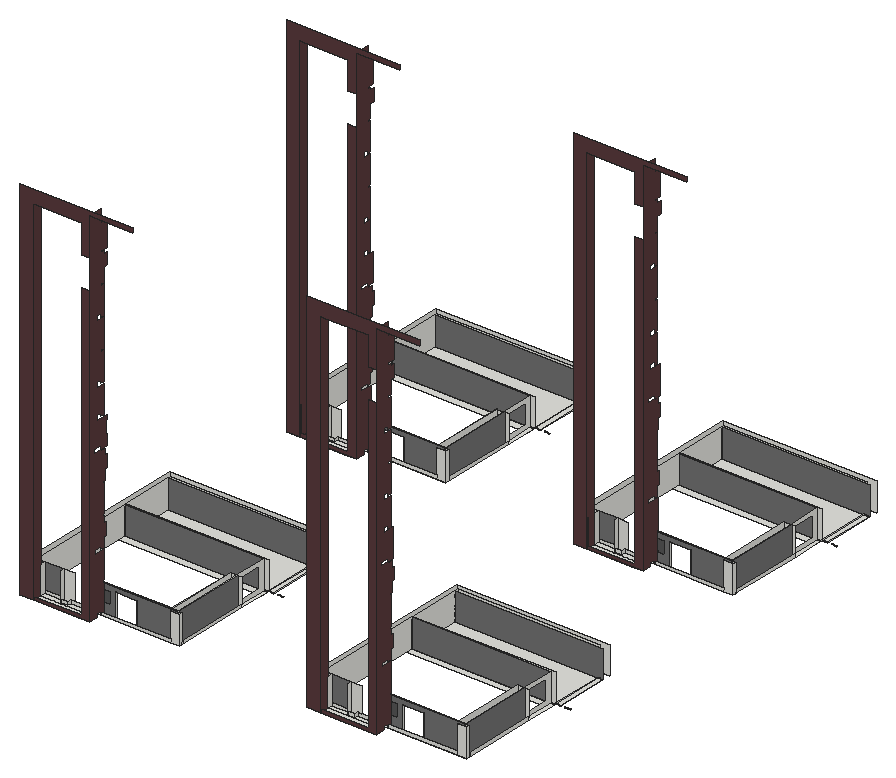
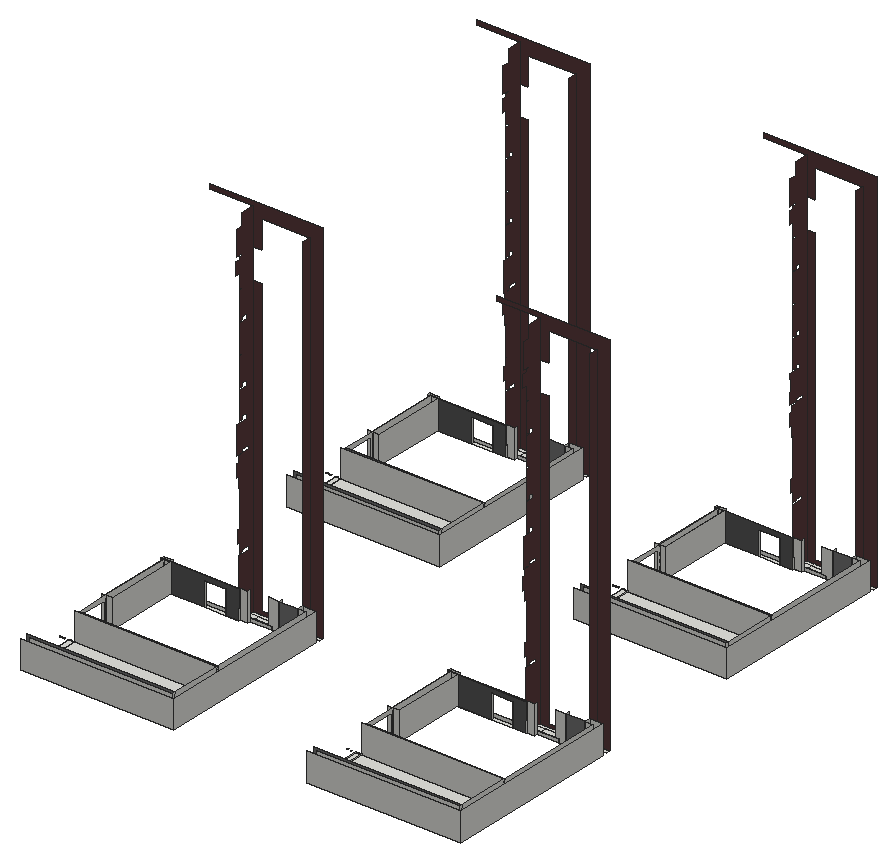
# SketchUp Ruby script. Lengths in inches.
U = 1.inch
M = Sketchup.active_model
def pt(a) = Geom::Point3d.new(a.map { |v| v * U })
def face(e, loops, mat)
  f = e.add_face(loops[0].map { |a| pt(a) })
  loops[1..].each { |l| e.add_face(l.map { |a| pt(a) }).erase! }
  f.material = f.back_material = mat if mat
  f
end
# faces: each face lists its corners as indices into pts; further lists are holes
def faces(e, pts, list, mat = nil) = list.each { |f| face(e, (f[0].is_a?(Array) ? f : [f]).map { |l| l.map { |i| pts[i] } }, mat) }
# xy, xz, yz: faces in a plane at the given z, y or x. An outline is a flat list of corners, or four numbers for a rectangle; further outlines are holes
def ring(l) = l.size == 4 ? [[l[0], l[1]], [l[2], l[1]], [l[2], l[3]], [l[0], l[3]]] : l.each_slice(2).to_a
def flat(e, list, mat, &to3) = list.each { |f| face(e, (f[0].is_a?(Array) ? f : [f]).map { |l| ring(l).map { |u, v| to3.(u, v) } }, mat) }
def xy(e, z, list, mat = nil) = flat(e, list, mat) { |x, y| [x, y, z] }
def xz(e, y, list, mat = nil) = flat(e, list, mat) { |x, z| [x, y, z] }
def yz(e, x, list, mat = nil) = flat(e, list, mat) { |y, z| [x, y, z] }
def lines(e, pts, list) = list.each { |a, b| e.add_line(pt(pts[a]), pt(pts[b])) }
# prism: a flat outline (further loops are holes) pulled along v
def prism(e, loops, v, mat = nil)
  f = face(e, loops, mat); d = Geom::Vector3d.new(v.map { |x| x * U })
  f.pushpull(f.normal.samedirection?(d) ? d.length : -d.length)
end
def box(e, o, s, mat = nil) = prism(e, [[o, [o[0] + s[0], o[1], o[2]], [o[0] + s[0], o[1] + s[1], o[2]], [o[0], o[1] + s[1], o[2]]]], [0, 0, s[2]], mat)
def at(x, y, z, deg = 0) = Geom::Transformation.translation(pt([x, y, z])) * Geom::Transformation.rotation(ORIGIN, Z_AXIS, deg.degrees)
def axes(o, x, y, z) = Geom::Transformation.new([*x, 0, *y, 0, *z, 0, *pt(o).to_a, 1])
def part(name) = M.definitions.add(name)
# library, detail: a bought-in or finely detailed component or shape, given as its bounding box
def library(name, o, s) = part(name).tap { |d| box(d.entities, o, s) }
def detail(e, o, s) = box(e.add_group.entities, o, s)
def put(e, d, t, mat = nil) = e.add_instance(d, t).tap { |i| i.material = mat if mat }
def group(e, t, mat = nil) = e.add_group.tap { |g| g.transformation = t; g.material = mat if mat }.entities
root = M.entities
M.materials.add("[Color M05]").color = [114, 114, 114]
M.materials.add("[Color M06]").color = [86, 86, 86]
M.materials.add("[Granite Brown]").color = [89, 59, 61]
xy(root,257.875,[[285.875,2258.18,890.875,2486.82],[1504.0625,2258.18,2109.0625,2486.82],[285.875,3672.87,890.875,3901.51],[1504.0625,3672.87,2109.0625,3901.51]])
xy(root,258,[[262.875,1763.25,319.53,1778.3125],[319.53,1763.25,523.04,1778.3125],[523.04,1763.25,557.88,1799.9375],[1481.0625,1763.25,1537.72,1778.3125],[1537.72,1763.25,1741.23,1778.3125],
  [1741.23,1763.25,1776.07,1799.9375],[319.53,1778.3125,523.04,1799.9375],[1537.72,1778.3125,1741.23,1799.9375],[319.53,1799.9375,523.04,1799.9375,523.04,1822.9375,431.33,1822.9375,431.33,1806.5625,399.91,1806.5625,399.91,1822.9375,319.53,1822.9375],[1537.72,1799.9375,1741.23,1799.9375,1741.23,1822.9375,1649.52,1822.9375,1649.52,1806.5625,1618.1,1806.5625,1618.1,1822.9375,1537.72,1822.9375],
  [523.04,1822.9375,557.88,1835.1875],[557.88,1822.9375,890.875,1822.9375,890.875,1835.1875,701.59,1835.1875,701.59,1839.6875,611.65,1839.6875,611.65,1835.1875,557.88,1835.1875],[1741.23,1822.9375,1776.07,1835.1875],[1776.07,1822.9375,2109.0625,1822.9375,2109.0625,1835.1875,1919.77,1835.1875,1919.77,1839.6875,1829.84,1839.6875,1829.84,1835.1875,1776.07,1835.1875],[557.4,1835.1875,611.65,1839.6875],
  [701.59,1835.1875,874.375,1839.6875],[874.375,1835.1875,890.875,1839.6875],[1775.59,1835.1875,1829.84,1839.6875],[1919.77,1835.1875,2092.5625,1839.6875],[2092.5625,1835.1875,2109.0625,1839.6875],
  [846.5625,1839.6875,847.0625,2148.83],[847.0625,1839.6875,874.375,2148.83],[874.375,1839.6875,878.5625,2148.83],[878.5625,1839.6875,890.875,2148.83],[2064.75,1839.6875,2065.25,2148.83],
  [2065.25,1839.6875,2092.5625,2148.83],[2092.5625,1839.6875,2096.75,2148.83],[2096.75,1839.6875,2109.0625,2148.83],[874.375,2148.83,890.875,2290],[2092.5625,2148.83,2109.0625,2290],
  [285.875,2290,890.875,2295.875],[1504.0625,2290,2109.0625,2295.875],[285.875,2295.875,890.875,2518.89],[890.875,2295.875,913.875,2518.89],[1504.0625,2295.875,2109.0625,2518.89],
  [2109.0625,2295.875,2132.0625,2518.89],[262.875,3177.9375,319.53,3193],[319.53,3177.9375,523.04,3193],[523.04,3177.9375,557.88,3214.625],[1481.0625,3177.9375,1537.72,3193],
  [1537.72,3177.9375,1741.23,3193],[1741.23,3177.9375,1776.07,3214.625],[319.53,3193,523.04,3214.625],[1537.72,3193,1741.23,3214.625],[319.53,3214.625,523.04,3214.625,523.04,3237.625,431.33,3237.625,431.33,3221.25,399.91,3221.25,399.91,3237.625,319.53,3237.625],
  [1537.72,3214.625,1741.23,3214.625,1741.23,3237.625,1649.52,3237.625,1649.52,3221.25,1618.1,3221.25,1618.1,3237.625,1537.72,3237.625],[523.04,3237.625,557.88,3249.875],[557.88,3237.625,890.875,3237.625,890.875,3249.875,701.59,3249.875,701.59,3254.375,611.65,3254.375,611.65,3249.875,557.88,3249.875],[1741.23,3237.625,1776.07,3249.875],[1776.07,3237.625,2109.0625,3237.625,2109.0625,3249.875,1919.77,3249.875,1919.77,3254.375,1829.84,3254.375,1829.84,3249.875,1776.07,3249.875],
  [557.4,3249.875,611.65,3254.375],[701.59,3249.875,874.375,3254.375],[874.375,3249.875,890.875,3254.375],[1775.59,3249.875,1829.84,3254.375],[1919.77,3249.875,2092.5625,3254.375],
  [2092.5625,3249.875,2109.0625,3254.375],[846.5625,3254.375,847.0625,3563.51],[847.0625,3254.375,874.375,3563.51],[874.375,3254.375,878.5625,3563.51],[878.5625,3254.375,890.875,3563.51],
  [2064.75,3254.375,2065.25,3563.51],[2065.25,3254.375,2092.5625,3563.51],[2092.5625,3254.375,2096.75,3563.51],[2096.75,3254.375,2109.0625,3563.51],[874.375,3563.51,890.875,3704.6875],
  [2092.5625,3563.51,2109.0625,3704.6875],[285.875,3704.6875,890.875,3710.5625],[1504.0625,3704.6875,2109.0625,3710.5625],[285.875,3710.5625,890.875,3933.57],[890.875,3710.5625,913.875,3933.57],
  [1504.0625,3710.5625,2109.0625,3933.57],[2109.0625,3710.5625,2132.0625,3933.57]])
xz(root,1763.25,[[262.875,258,319.53,258,319.53,1764,523.04,1764,523.04,1644,557.88,1644,557.88,1764,557.22,1764,557.22,1805.3125,557.4,1805.3125,557.4,1801.625,741.54,1801.625,741.54,1821.625,262.875,1821.625],[319.53,258,557.88,258,557.88,1518,523.04,1518,523.04,271.9375,320.25,271.9375,320.25,378,319.53,378],[1481.0625,258,1537.72,258,1537.72,1764,1741.23,1764,1741.23,1644,1776.07,1644,1776.07,1764,1775.4,1764,1775.4,1805.3125,1775.59,1805.3125,1775.59,1801.625,1959.73,1801.625,1959.73,1821.625,1481.0625,1821.625],[1537.72,258,1776.07,258,1776.07,1518,1741.23,1518,1741.23,271.9375,1538.44,271.9375,1538.44,378,1537.72,378]],"[Granite Brown]")
xz(root,1799.9375,[[262.875,258,319.53,378],[1481.0625,258,1537.72,378]])
xz(root,1806.5625,[[399.91,258,399.91,271.9375,399.98,271.9375],[399.91,258,431.33,258,431.33,271.9375,399.98,271.9375],[1618.1,258,1618.1,271.9375,1618.17,271.9375],[1618.1,258,1649.52,258,1649.52,271.9375,1618.17,271.9375]])
xz(root,1822.9375,[[285.875,258,319.53,378],[319.53,258,399.91,258,399.91,271.9375,320.25,271.9375,320.25,378,319.53,378],[399.91,258,400.51,378,445.4,378,445.4,271.9375,431.33,271.9375,431.33,258],[431.33,258,523.04,271.9375],[557.88,258,852.75,272.125],
  [852.75,258,890.875,377],[1504.0625,258,1537.72,378],[1537.72,258,1618.1,258,1618.1,271.9375,1538.44,271.9375,1538.44,378,1537.72,378],[1618.1,258,1618.7,378,1663.58,378,1663.58,271.9375,1649.52,271.9375,1649.52,258],[1649.52,258,1741.23,271.9375],
  [1776.07,258,2070.9375,272.125],[2070.9375,258,2109.0625,377]])
xz(root,1822.9375,[[399.91,258,400.51,378,320.25,378,320.25,271.9375,399.91,271.9375],[1618.1,258,1618.7,378,1538.44,378,1538.44,271.9375,1618.1,271.9375]],"[Color M05]")
xz(root,1835.1875,[[523.04,258,557.4,378],[874.375,258,890.875,377],[1741.23,258,1775.59,378],[2092.5625,258,2109.0625,377]])
xz(root,1835.1875,[[557.88,258,611.65,258,611.65,358.625,701.59,358.625,701.59,258,874.375,258,874.375,377,557.88,377,557.88,354.03,589.71,354.03,589.71,301.74,557.88,301.74],[1776.07,258,1829.84,258,1829.84,358.625,1919.77,358.625,1919.77,258,2092.5625,258,2092.5625,377,1776.07,377,1776.07,354.03,1807.9,354.03,1807.9,301.74,1776.07,301.74]],"[Color M05]")
xz(root,1835.1875,[[557.4,258,557.88,301.74],[1775.59,258,1776.07,301.74]],"[Granite Brown]")
xz(root,1839.6875,[[846.5625,258,847.0625,378],[847.0625,258,874.375,378],[874.375,258,878.5625,378],[2064.75,258,2065.25,378],[2065.25,258,2092.5625,378],
  [2092.5625,258,2096.75,378]])
xz(root,1839.6875,[[557.4,258,557.4,378,846.5625,378,846.5625,258,701.59,258,701.59,358.625,611.65,358.625,611.65,258],[1775.59,258,1775.59,378,2064.75,378,2064.75,258,1919.77,258,1919.77,358.625,1829.84,358.625,1829.84,258]],"[Color M06]")
xz(root,2148.83,[[846.5625,258,847.0625,378],[847.0625,258,874.375,378],[874.375,258,878.5625,378],[878.5625,258,890.875,258,890.875,271.5,894.3125,271.5,894.3125,378,878.5625,378],[2064.75,258,2065.25,378],
  [2065.25,258,2092.5625,378],[2092.5625,258,2096.75,378],[2096.75,258,2109.0625,258,2109.0625,271.5,2112.5,271.5,2112.5,378,2096.75,378]])
xz(root,2290,[[874.375,258,890.875,259.75],[2092.5625,258,2109.0625,259.75]])
xz(root,2290,[[285.875,258,874.375,378],[1504.0625,258,2092.5625,378]],"[Color M05]")
xz(root,2295.875,[[285.875,258,890.875,378],[890.875,258,913.875,259.75],[930.75,258,954.6875,259.75],[1504.0625,258,2109.0625,378],[2109.0625,258,2132.0625,259.75],
  [2148.9375,258,2172.875,259.75]])
xz(root,2518.89,[[890.875,258,913.875,259.75],[2109.0625,258,2132.0625,259.75]])
xz(root,2518.89,[[285.875,258,890.875,258,890.875,259.75,913.875,259.75,913.875,378,285.875,378],[1504.0625,258,2109.0625,258,2109.0625,259.75,2132.0625,259.75,2132.0625,378,1504.0625,378]],"[Color M05]")
xz(root,2531.375,[[285.875,258,890.875,378],[1504.0625,258,2109.0625,378]])
xz(root,2554.375,[[262.875,258,913.875,378],[1481.0625,258,2132.0625,378]])
xz(root,3177.9375,[[262.875,258,319.53,258,319.53,1764,523.04,1764,523.04,1644,557.88,1644,557.88,1764,557.22,1764,557.22,1805.3125,557.4,1805.3125,557.4,1801.625,741.54,1801.625,741.54,1821.625,262.875,1821.625],[319.53,258,557.88,258,557.88,1518,523.04,1518,523.04,271.9375,320.25,271.9375,320.25,378,319.53,378],[1481.0625,258,1537.72,258,1537.72,1764,1741.23,1764,1741.23,1644,1776.07,1644,1776.07,1764,1775.4,1764,1775.4,1805.3125,1775.59,1805.3125,1775.59,1801.625,1959.73,1801.625,1959.73,1821.625,1481.0625,1821.625],[1537.72,258,1776.07,258,1776.07,1518,1741.23,1518,1741.23,271.9375,1538.44,271.9375,1538.44,378,1537.72,378]],"[Granite Brown]")
xz(root,3214.625,[[262.875,258,319.53,378],[1481.0625,258,1537.72,378]])
xz(root,3221.25,[[399.91,258,399.91,271.9375,399.98,271.9375],[399.91,258,431.33,258,431.33,271.9375,399.98,271.9375],[1618.1,258,1618.1,271.9375,1618.17,271.9375],[1618.1,258,1649.52,258,1649.52,271.9375,1618.17,271.9375]])
xz(root,3237.625,[[285.875,258,319.53,378],[319.53,258,399.91,258,399.91,271.9375,320.25,271.9375,320.25,378,319.53,378],[399.91,258,400.51,378,445.4,378,445.4,271.9375,431.33,271.9375,431.33,258],[431.33,258,523.04,271.9375],[557.88,258,852.75,272.125],
  [852.75,258,890.875,377],[1504.0625,258,1537.72,378],[1537.72,258,1618.1,258,1618.1,271.9375,1538.44,271.9375,1538.44,378,1537.72,378],[1618.1,258,1618.7,378,1663.58,378,1663.58,271.9375,1649.52,271.9375,1649.52,258],[1649.52,258,1741.23,271.9375],
  [1776.07,258,2070.9375,272.125],[2070.9375,258,2109.0625,377]])
xz(root,3237.625,[[399.91,258,400.51,378,320.25,378,320.25,271.9375,399.91,271.9375],[1618.1,258,1618.7,378,1538.44,378,1538.44,271.9375,1618.1,271.9375]],"[Color M05]")
xz(root,3249.875,[[523.04,258,557.4,378],[874.375,258,890.875,377],[1741.23,258,1775.59,378],[2092.5625,258,2109.0625,377]])
xz(root,3249.875,[[557.88,258,611.65,258,611.65,358.625,701.59,358.625,701.59,258,874.375,258,874.375,377,557.88,377,557.88,354.03,589.71,354.03,589.71,301.74,557.88,301.74],[1776.07,258,1829.84,258,1829.84,358.625,1919.77,358.625,1919.77,258,2092.5625,258,2092.5625,377,1776.07,377,1776.07,354.03,1807.9,354.03,1807.9,301.74,1776.07,301.74]],"[Color M05]")
xz(root,3249.875,[[557.4,258,557.88,301.74],[1775.59,258,1776.07,301.74]],"[Granite Brown]")
xz(root,3254.375,[[846.5625,258,847.0625,378],[847.0625,258,874.375,378],[874.375,258,878.5625,378],[2064.75,258,2065.25,378],[2065.25,258,2092.5625,378],
  [2092.5625,258,2096.75,378]])
xz(root,3254.375,[[557.4,258,557.4,378,846.5625,378,846.5625,258,701.59,258,701.59,358.625,611.65,358.625,611.65,258],[1775.59,258,1775.59,378,2064.75,378,2064.75,258,1919.77,258,1919.77,358.625,1829.84,358.625,1829.84,258]],"[Color M06]")
xz(root,3563.51,[[846.5625,258,847.0625,378],[847.0625,258,874.375,378],[874.375,258,878.5625,378],[878.5625,258,890.875,258,890.875,271.5,894.3125,271.5,894.3125,378,878.5625,378],[2064.75,258,2065.25,378],
  [2065.25,258,2092.5625,378],[2092.5625,258,2096.75,378],[2096.75,258,2109.0625,258,2109.0625,271.5,2112.5,271.5,2112.5,378,2096.75,378]])
xz(root,3704.6875,[[874.375,258,890.875,259.75],[2092.5625,258,2109.0625,259.75]])
xz(root,3704.6875,[[285.875,258,874.375,378],[1504.0625,258,2092.5625,378]],"[Color M05]")
xz(root,3710.5625,[[285.875,258,890.875,378],[890.875,258,913.875,259.75],[930.75,258,954.6875,259.75],[1504.0625,258,2109.0625,378],[2109.0625,258,2132.0625,259.75],
  [2148.9375,258,2172.875,259.75]])
xz(root,3933.57,[[890.875,258,913.875,259.75],[2109.0625,258,2132.0625,259.75]])
xz(root,3933.57,[[285.875,258,890.875,258,890.875,259.75,913.875,259.75,913.875,378,285.875,378],[1504.0625,258,2109.0625,258,2109.0625,259.75,2132.0625,259.75,2132.0625,378,1504.0625,378]],"[Color M05]")
xz(root,3946.0625,[[285.875,258,890.875,378],[1504.0625,258,2109.0625,378]])
xz(root,3969.0625,[[262.875,258,913.875,378],[1481.0625,258,2132.0625,378]])
yz(root,262.875,[[1799.9375,258,2554.375,378],[3214.625,258,3969.0625,378]])
yz(root,285.875,[[1822.9375,258,2290,378],[2290,258,2295.875,378],[2295.875,258,2518.89,378],[2518.89,258,2531.375,378],[3237.625,258,3704.6875,378],
  [3704.6875,258,3710.5625,378],[3710.5625,258,3933.57,378],[3933.57,258,3946.0625,378]])
yz(root,319.53,[[1799.9375,258,1822.9375,378],[3214.625,258,3237.625,378]])
yz(root,319.53,[[1763.25,258,1799.9375,1764],[3177.9375,258,3214.625,1764]],"[Granite Brown]")
yz(root,399.91,[[1806.5625,258,1822.9375,271.9375],[3221.25,258,3237.625,271.9375]])
yz(root,431.33,[[1806.5625,258,1822.9375,271.9375],[3221.25,258,3237.625,271.9375]])
yz(root,523.04,[[1822.9375,258,1835.1875,378],[3237.625,258,3249.875,378]])
yz(root,557.4,[[1835.1875,258,1839.6875,301.74],[3249.875,258,3254.375,301.74]])
yz(root,557.88,[[1763.25,258,1799.9375,258,1799.9375,272.125,1822.9375,272.125,1822.9375,258,1835.1875,258,1835.1875,377,1834.0625,377,1834.0625,384,1837.8125,384,1837.8125,504,1788.5,504,1788.5,517.25,1822.9375,517.25,1822.9375,510,1835.1875,510,1835.1875,551.24,1845.8125,551.24,1845.8125,603.53,1835.1875,603.53,1835.1875,630,1833.5,630,1833.5,636,1835.1875,636,1835.1875,756,1833.5,756,1833.5,762,1842.5,762,1842.5,805.12,1853.125,805.12,1853.125,857.4,1842.5,857.4,1842.5,882,1822.9375,882,1822.9375,888,1786.97,888,1786.97,900.6875,1822.9375,900.6875,1822.9375,888,1850.9375,888,1850.9375,934.68,1848.875,934.68,1848.875,986.96,1850.9375,986.96,1850.9375,1008,1799.9375,1008,1799.9375,1026.6875,1822.9375,1026.6875,1822.9375,1014,1835.1875,1014,1835.1875,1134,1799.9375,1134,1799.9375,1152.6875,1822.9375,1152.6875,1822.9375,1140,1835.1875,1140,1835.1875,1260,1822.9375,1260,1822.9375,1266,1835.1875,1266,1835.1875,1386,1799.9375,1386,1799.9375,1404.6875,1822.9375,1404.6875,1822.9375,1392,1835.1875,1392,1835.1875,1512,1822.9375,1512,1822.9375,1518,1835.1875,1518,1835.1875,1575.17,1854.3125,1575.17,1854.3125,1627.45,1835.1875,1627.45,1835.1875,1638,1822.9375,1638,1822.9375,1644,1851.6875,1644,1851.6875,1749.375,1822.9375,1749.375,1822.9375,1801.625,1763.25,1801.625],[3177.9375,258,3214.625,258,3214.625,272.125,3237.625,272.125,3237.625,258,3249.875,258,3249.875,377,3248.75,377,3248.75,384,3252.5,384,3252.5,504,3203.1875,504,3203.1875,517.25,3237.625,517.25,3237.625,510,3249.875,510,3249.875,551.24,3260.5,551.24,3260.5,603.53,3249.875,603.53,3249.875,630,3248.1875,630,3248.1875,636,3249.875,636,3249.875,756,3248.1875,756,3248.1875,762,3257.1875,762,3257.1875,805.12,3267.8125,805.12,3267.8125,857.4,3257.1875,857.4,3257.1875,882,3237.625,882,3237.625,888,3201.66,888,3201.66,900.6875,3237.625,900.6875,3237.625,888,3265.625,888,3265.625,934.68,3263.5625,934.68,3263.5625,986.96,3265.625,986.96,3265.625,1008,3214.625,1008,3214.625,1026.6875,3237.625,1026.6875,3237.625,1014,3249.875,1014,3249.875,1134,3214.625,1134,3214.625,1152.6875,3237.625,1152.6875,3237.625,1140,3249.875,1140,3249.875,1260,3237.625,1260,3237.625,1266,3249.875,1266,3249.875,1386,3214.625,1386,3214.625,1404.6875,3237.625,1404.6875,3237.625,1392,3249.875,1392,3249.875,1512,3237.625,1512,3237.625,1518,3249.875,1518,3249.875,1575.17,3269,1575.17,3269,1627.45,3249.875,1627.45,3249.875,1638,3237.625,1638,3237.625,1644,3266.375,1644,3266.375,1749.375,3237.625,1749.375,3237.625,1801.625,3177.9375,1801.625]],"[Granite Brown]")
yz(root,611.65,[[1835.1875,258,1839.6875,358.625],[3249.875,258,3254.375,358.625]])
yz(root,701.59,[[1835.1875,258,1839.6875,358.625],[3249.875,258,3254.375,358.625]])
yz(root,846.5625,[[1839.6875,258,2148.83,378],[3254.375,258,3563.51,378]])
yz(root,847.0625,[[1839.6875,258,2148.83,378],[3254.375,258,3563.51,378]])
yz(root,874.375,[[1835.1875,258,1839.6875,378],[1839.6875,258,2148.83,378],[[2148.83,258,2290,378],[2156.01,275.36,2266.33,361.04]],[3249.875,258,3254.375,378],[3254.375,258,3563.51,378],
  [[3563.51,258,3704.6875,378],[3570.7,275.36,3681.01,361.04]]])
yz(root,878.5625,[[1839.6875,258,2148.83,378],[3254.375,258,3563.51,378]],"[Color M05]")
yz(root,890.875,[[1822.9375,258,1835.1875,377],[1835.1875,258,1839.6875,271.5],[1839.6875,258,2148.83,271.5],[2290,258,2295.875,259.75],[2295.875,258,2518.89,259.75],
  [3237.625,258,3249.875,377],[3249.875,258,3254.375,271.5],[3254.375,258,3563.51,271.5],[3704.6875,258,3710.5625,259.75],[3710.5625,258,3933.57,259.75]])
yz(root,913.875,[[2295.875,258,2518.89,259.75],[3710.5625,258,3933.57,259.75]])
yz(root,1481.0625,[[1799.9375,258,2554.375,378],[3214.625,258,3969.0625,378]])
yz(root,1504.0625,[[1822.9375,258,2290,378],[2290,258,2295.875,378],[2295.875,258,2518.89,378],[2518.89,258,2531.375,378],[3237.625,258,3704.6875,378],
  [3704.6875,258,3710.5625,378],[3710.5625,258,3933.57,378],[3933.57,258,3946.0625,378]])
yz(root,1537.72,[[1799.9375,258,1822.9375,378],[3214.625,258,3237.625,378]])
yz(root,1537.72,[[1763.25,258,1799.9375,1764],[3177.9375,258,3214.625,1764]],"[Granite Brown]")
yz(root,1618.1,[[1806.5625,258,1822.9375,271.9375],[3221.25,258,3237.625,271.9375]])
yz(root,1649.52,[[1806.5625,258,1822.9375,271.9375],[3221.25,258,3237.625,271.9375]])
yz(root,1741.23,[[1822.9375,258,1835.1875,378],[3237.625,258,3249.875,378]])
yz(root,1775.59,[[1835.1875,258,1839.6875,301.74],[3249.875,258,3254.375,301.74]])
yz(root,1776.07,[[1763.25,258,1799.9375,258,1799.9375,272.125,1822.9375,272.125,1822.9375,258,1835.1875,258,1835.1875,377,1834.0625,377,1834.0625,384,1837.8125,384,1837.8125,504,1788.5,504,1788.5,517.25,1822.9375,517.25,1822.9375,510,1835.1875,510,1835.1875,551.24,1845.8125,551.24,1845.8125,603.53,1835.1875,603.53,1835.1875,630,1833.5,630,1833.5,636,1835.1875,636,1835.1875,756,1833.5,756,1833.5,762,1842.5,762,1842.5,805.12,1853.125,805.12,1853.125,857.4,1842.5,857.4,1842.5,882,1822.9375,882,1822.9375,888,1786.97,888,1786.97,900.6875,1822.9375,900.6875,1822.9375,888,1850.9375,888,1850.9375,934.68,1848.875,934.68,1848.875,986.96,1850.9375,986.96,1850.9375,1008,1799.9375,1008,1799.9375,1026.6875,1822.9375,1026.6875,1822.9375,1014,1835.1875,1014,1835.1875,1134,1799.9375,1134,1799.9375,1152.6875,1822.9375,1152.6875,1822.9375,1140,1835.1875,1140,1835.1875,1260,1822.9375,1260,1822.9375,1266,1835.1875,1266,1835.1875,1386,1799.9375,1386,1799.9375,1404.6875,1822.9375,1404.6875,1822.9375,1392,1835.1875,1392,1835.1875,1512,1822.9375,1512,1822.9375,1518,1835.1875,1518,1835.1875,1575.17,1854.3125,1575.17,1854.3125,1627.45,1835.1875,1627.45,1835.1875,1638,1822.9375,1638,1822.9375,1644,1851.6875,1644,1851.6875,1749.375,1822.9375,1749.375,1822.9375,1801.625,1763.25,1801.625],[3177.9375,258,3214.625,258,3214.625,272.125,3237.625,272.125,3237.625,258,3249.875,258,3249.875,377,3248.75,377,3248.75,384,3252.5,384,3252.5,504,3203.1875,504,3203.1875,517.25,3237.625,517.25,3237.625,510,3249.875,510,3249.875,551.24,3260.5,551.24,3260.5,603.53,3249.875,603.53,3249.875,630,3248.1875,630,3248.1875,636,3249.875,636,3249.875,756,3248.1875,756,3248.1875,762,3257.1875,762,3257.1875,805.12,3267.8125,805.12,3267.8125,857.4,3257.1875,857.4,3257.1875,882,3237.625,882,3237.625,888,3201.66,888,3201.66,900.6875,3237.625,900.6875,3237.625,888,3265.625,888,3265.625,934.68,3263.5625,934.68,3263.5625,986.96,3265.625,986.96,3265.625,1008,3214.625,1008,3214.625,1026.6875,3237.625,1026.6875,3237.625,1014,3249.875,1014,3249.875,1134,3214.625,1134,3214.625,1152.6875,3237.625,1152.6875,3237.625,1140,3249.875,1140,3249.875,1260,3237.625,1260,3237.625,1266,3249.875,1266,3249.875,1386,3214.625,1386,3214.625,1404.6875,3237.625,1404.6875,3237.625,1392,3249.875,1392,3249.875,1512,3237.625,1512,3237.625,1518,3249.875,1518,3249.875,1575.17,3269,1575.17,3269,1627.45,3249.875,1627.45,3249.875,1638,3237.625,1638,3237.625,1644,3266.375,1644,3266.375,1749.375,3237.625,1749.375,3237.625,1801.625,3177.9375,1801.625]],"[Granite Brown]")
yz(root,1829.84,[[1835.1875,258,1839.6875,358.625],[3249.875,258,3254.375,358.625]])
yz(root,1919.77,[[1835.1875,258,1839.6875,358.625],[3249.875,258,3254.375,358.625]])
yz(root,2064.75,[[1839.6875,258,2148.83,378],[3254.375,258,3563.51,378]])
yz(root,2065.25,[[1839.6875,258,2148.83,378],[3254.375,258,3563.51,378]])
yz(root,2092.5625,[[1835.1875,258,1839.6875,378],[1839.6875,258,2148.83,378],[[2148.83,258,2290,378],[2156.01,275.36,2266.33,361.04]],[3249.875,258,3254.375,378],[3254.375,258,3563.51,378],
  [[3563.51,258,3704.6875,378],[3570.7,275.36,3681.01,361.04]]])
yz(root,2096.75,[[1839.6875,258,2148.83,378],[3254.375,258,3563.51,378]],"[Color M05]")
yz(root,2109.0625,[[1822.9375,258,1835.1875,377],[1835.1875,258,1839.6875,271.5],[1839.6875,258,2148.83,271.5],[2290,258,2295.875,259.75],[2295.875,258,2518.89,259.75],
  [3237.625,258,3249.875,377],[3249.875,258,3254.375,271.5],[3254.375,258,3563.51,271.5],[3704.6875,258,3710.5625,259.75],[3710.5625,258,3933.57,259.75]])
yz(root,2132.0625,[[2295.875,258,2518.89,259.75],[3710.5625,258,3933.57,259.75]])
p = [[399.91,1822.9375,258],[399.91,1806.5625,258],[399.98,1806.5625,271.9375],[400.51,1806.5625,378],[400.51,1822.9375,378],[1618.1,1822.9375,258],
  [1618.1,1806.5625,258],[1618.17,1806.5625,271.9375],[1618.7,1806.5625,378],[1618.7,1822.9375,378],[399.91,3237.625,258],[399.91,3221.25,258],
  [399.98,3221.25,271.9375],[400.51,3221.25,378],[400.51,3237.625,378],[1618.1,3237.625,258],[1618.1,3221.25,258],[1618.17,3221.25,271.9375],
  [1618.7,3221.25,378],[1618.7,3237.625,378],[1741.23,1778.3125,258],[1775.59,1778.3125,258],[523.04,1778.3125,258],[557.4,1778.3125,258],
  [1741.23,3193,258],[1775.59,3193,258],[523.04,3193,258],[557.4,3193,258]]
faces(root,p,[[0,1,2,3,4],[5,6,7,8,9],[10,11,12,13,14],[15,16,17,18,19]])
lines(root,p,[[20,21],[22,23],[24,25],[26,27]])
